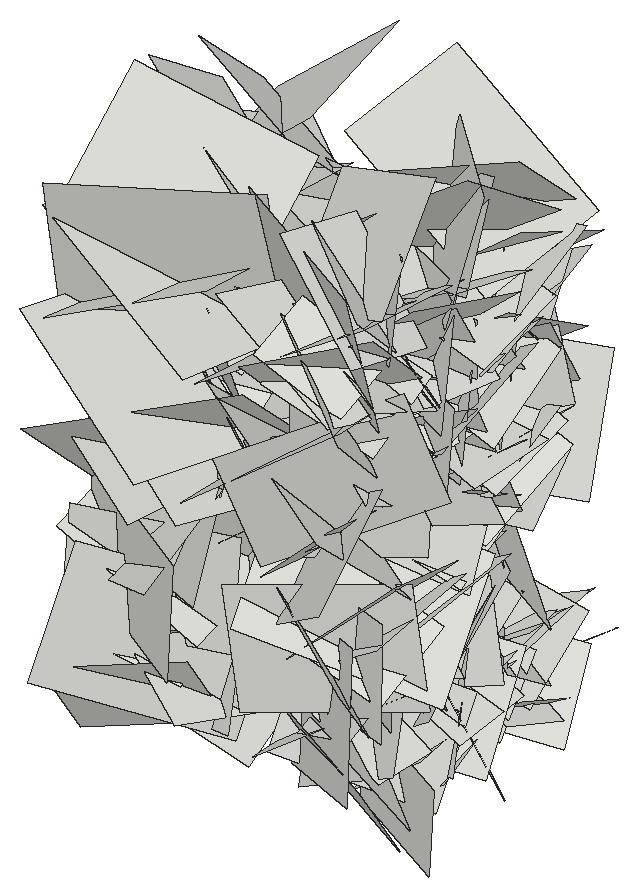
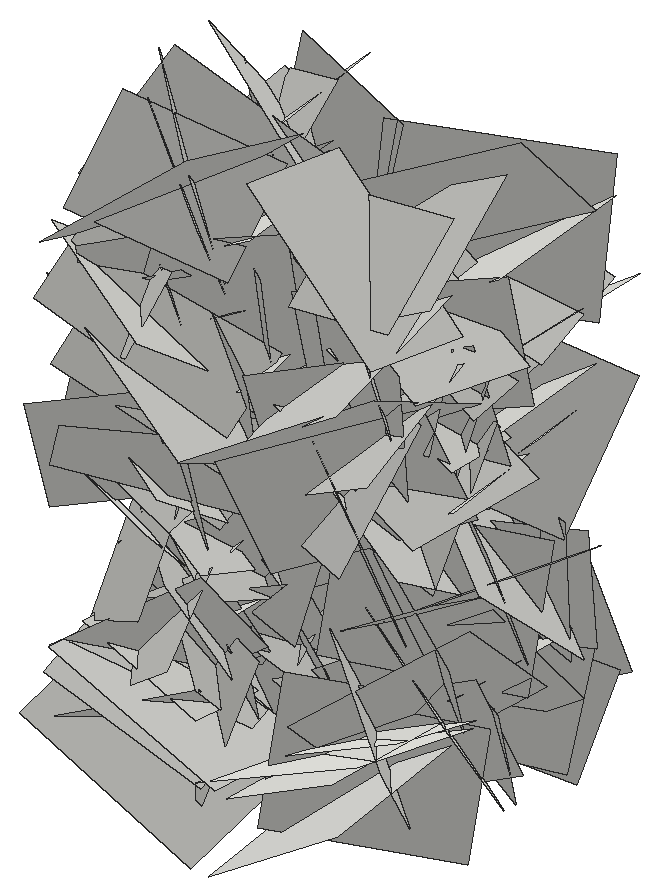
# SketchUp Ruby script. Lengths in inches.
U = 1.inch
M = Sketchup.active_model
def pt(a) = Geom::Point3d.new(a.map { |v| v * U })
def face(e, loops, mat)
  f = e.add_face(loops[0].map { |a| pt(a) })
  loops[1..].each { |l| e.add_face(l.map { |a| pt(a) }).erase! }
  f.material = f.back_material = mat if mat
  f
end
# faces: each face lists its corners as indices into pts; further lists are holes
def faces(e, pts, list, mat = nil) = list.each { |f| face(e, (f[0].is_a?(Array) ? f : [f]).map { |l| l.map { |i| pts[i] } }, mat) }
# xy, xz, yz: faces in a plane at the given z, y or x. An outline is a flat list of corners, or four numbers for a rectangle; further outlines are holes
def ring(l) = l.size == 4 ? [[l[0], l[1]], [l[2], l[1]], [l[2], l[3]], [l[0], l[3]]] : l.each_slice(2).to_a
def flat(e, list, mat, &to3) = list.each { |f| face(e, (f[0].is_a?(Array) ? f : [f]).map { |l| ring(l).map { |u, v| to3.(u, v) } }, mat) }
def xy(e, z, list, mat = nil) = flat(e, list, mat) { |x, y| [x, y, z] }
def xz(e, y, list, mat = nil) = flat(e, list, mat) { |x, z| [x, y, z] }
def yz(e, x, list, mat = nil) = flat(e, list, mat) { |y, z| [x, y, z] }
def lines(e, pts, list) = list.each { |a, b| e.add_line(pt(pts[a]), pt(pts[b])) }
# prism: a flat outline (further loops are holes) pulled along v
def prism(e, loops, v, mat = nil)
  f = face(e, loops, mat); d = Geom::Vector3d.new(v.map { |x| x * U })
  f.pushpull(f.normal.samedirection?(d) ? d.length : -d.length)
end
def box(e, o, s, mat = nil) = prism(e, [[o, [o[0] + s[0], o[1], o[2]], [o[0] + s[0], o[1] + s[1], o[2]], [o[0], o[1] + s[1], o[2]]]], [0, 0, s[2]], mat)
def at(x, y, z, deg = 0) = Geom::Transformation.translation(pt([x, y, z])) * Geom::Transformation.rotation(ORIGIN, Z_AXIS, deg.degrees)
def axes(o, x, y, z) = Geom::Transformation.new([*x, 0, *y, 0, *z, 0, *pt(o).to_a, 1])
def part(name) = M.definitions.add(name)
# library, detail: a bought-in or finely detailed component or shape, given as its bounding box
def library(name, o, s) = part(name).tap { |d| box(d.entities, o, s) }
def detail(e, o, s) = box(e.add_group.entities, o, s)
def put(e, d, t, mat = nil) = e.add_instance(d, t).tap { |i| i.material = mat if mat }
def group(e, t, mat = nil) = e.add_group.tap { |g| g.transformation = t; g.material = mat if mat }.entities
root = M.entities
c1 = part("Component\#6")
p = [[0.01,0,0],[0,3.24,4.54],[4.32,3.24,4.54],[4.33,0,0]]
faces(c1.entities,p,[[0,1,2,3]])
put(root,c1,axes([400.91,196.19,13.89],[-0.03711,0.95345,-0.08325],[0.1071,-0.07916,-0.94908],[1.00884,0.04348,0.09769]))
put(root,c1,axes([404.88,198.53,13.8],[0.10676,-0.41647,0.70694],[0.09382,0.7136,0.40779],[-0.86465,0.02601,0.13154]))
put(root,c1,axes([404.88,201.03,8.02],[0.03451,-0.61291,-0.20918],[-0.0475,-0.21108,0.61149],[-0.68484,-0.01625,-0.05296]))
put(root,c1,axes([404.88,199.53,17.66],[0.07108,0.22718,0.77768],[0.14032,0.76678,-0.23541],[-0.84726,0.14605,0.02626]))
put(root,c1,axes([404.88,196.1,5.28],[0.08762,-0.56519,-0.39893],[-0.0287,-0.4041,0.56691],[-0.73275,-0.05175,-0.06991]))
put(root,c1,axes([400.91,192.44,8.79],[-0.05887,1.04295,0.25043],[0.00297,0.2509,-1.04431],[1.13694,0.05335,0.0157]))
put(root,c1,axes([400.91,193.71,0.46],[0.00413,-0.52236,0.7551],[0.18121,0.74232,0.51263],[0.95624,-0.13842,-0.10041]))
put(root,c1,axes([400.91,195.28,4.79],[0.03702,0.87634,0.85063],[-0.28559,0.83554,-0.84973],[1.26267,0.16329,-0.21713]))
put(root,c1,axes([400.91,203.91,5.3125],[0.18463,-0.58129,-0.78091],[-0.13848,-0.80009,0.56643],[1.02258,-0.00339,0.2177]))
put(root,c1,axes([400.91,198.93,5.125],[0.08676,0.85287,0.14934],[0.16568,0.13299,-0.84515],[0.90272,-0.10637,0.14076]))
put(root,c1,axes([400.91,198.84,9.75],[-0.24721,-0.9594,-0.88495],[-0.06038,-0.89063,0.98057],[1.38221,-0.2105,-0.11544]))
put(root,c1,axes([400.91,202.1,18.26],[-0.1919,-1.13475,-0.09678],[0.16378,-0.12156,1.13628],[1.19604,-0.16542,-0.17113]))
put(root,c1,axes([404.88,194.11,10.49],[0.01019,-0.66626,0.06574],[0.1187,0.06642,0.65679],[-0.69967,0.00157,0.11238]))
put(root,c1,axes([400.91,200.51,5.45],[-0.07717,-0.59417,-0.91785],[0.09928,-0.91989,0.58806],[1.15472,0.03938,-0.1119]))
put(root,c1,axes([400.91,205.24,14.9],[-0.1168,-0.46047,-1.13614],[-0.0362,-1.13913,0.465],[1.29896,-0.07315,-0.0892]))
put(root,c1,axes([400.91,194.25,1.05],[0.1707,-0.55728,0.79671],[-0.04122,0.80323,0.5697],[1.02978,0.12452,-0.10926]))
put(root,c1,axes([400.91,194.35,10.5],[-0.1187,0.07765,-1.12146],[0.14385,-1.11784,-0.09095],[1.18288,0.14373,-0.10148]))
put(root,c1,axes([400.91,197.36,24.8],[-0.09794,1.0389,-0.68546],[-0.01654,-0.68826,-1.04104],[1.31923,0.0685,-0.06394]))
put(root,c1,axes([404.88,199.74,12.37],[0.13977,-0.41949,-0.41774],[-0.0557,-0.43458,0.41982],[-0.62506,-0.05508,-0.13082]))
put(root,c1,axes([404.88,199.42,15.6],[0.03605,-0.49998,-0.38134],[0.14474,-0.36691,0.49324],[-0.65063,-0.10932,0.0886]))
put(root,c1,axes([400.91,200.08,24.34],[0.03463,0.75517,-0.67877],[0.20748,-0.67107,-0.73718],[1.05612,0.10708,0.16708]))
put(root,c1,axes([400.91,199.09,16.39],[0.13116,-1.14374,0.05938],[-0.13174,0.04596,1.1443],[1.20683,0.12933,0.11846]))
put(root,c1,axes([400.91,192.66,5.0625],[0.03803,0.06475,1.02957],[0.25075,1.00223,-0.07127],[1.06436,-0.23842,-0.02]))
put(root,c1,axes([400.91,196.53,2.03],[0.14871,0.38131,0.94323],[0.09041,0.94439,-0.39446],[1.07463,-0.13222,-0.09734]))
put(root,c1,axes([400.91,200.2,14.91],[0.20407,-0.96139,-0.18597],[0.07393,-0.17559,0.97991],[1.03533,0.20204,-0.03331]))
put(root,c1,axes([400.91,198.375,11.05],[-0.00636,-0.47599,-1.14741],[-0.03555,-1.14695,0.47597],[1.31628,-0.03327,0.00731]))
put(root,c1,axes([400.91,202.25,12.93],[-0.19135,-1.27912,0.12446],[0.2118,0.09622,1.27869],[1.34571,-0.19703,-0.18355]))
put(root,c1,axes([400.91,197.86,18.23],[0.19608,0.2602,-1.0463],[-0.01915,-1.06069,-0.26697],[1.14269,-0.06243,0.17507]))
put(root,c1,axes([400.91,197.84,4.84],[0.11369,-0.36766,-0.96616],[0.19069,-0.94989,0.38144],[1.07906,0.2066,0.03439]))
put(root,c1,axes([400.91,200.375,7.61],[0.26418,-0.51362,-0.84712],[0.05211,-0.86603,0.53955],[1.04881,0.1724,0.18657]))
put(root,c1,axes([400.91,203.04,12.11],[0.14841,-0.94408,-0.5752],[0.05434,-0.57362,0.95398],[1.17058,0.14632,0.02864]))
put(root,c1,axes([400.91,199.56,18.73],[0.07364,1.07871,-0.62029],[-0.05176,-0.61841,-1.08091],[1.31797,-0.08456,-0.00779]))
put(root,c1,axes([400.91,204.42,20.53],[0.1154,-1.25003,-0.28156],[-0.14973,-0.29256,1.24425],[1.34995,0.07441,0.16208]))
put(root,c1,axes([400.91,195.93,15.54],[0.04965,0.25406,1.2028],[0.02984,1.20314,-0.25523],[1.30276,-0.03724,-0.03999]))
put(root,c1,axes([400.91,198.85,12.57],[0.15345,0.48368,1.12599],[-0.09378,1.13498,-0.47617],[1.29562,0.02486,-0.16783]))
put(root,c1,axes([400.91,200.7,5.85],[0.20906,1.0682,-0.14016],[0.07965,-0.15578,-1.08152],[1.13921,-0.18514,0.10133]))
put(root,c1,axes([400.91,194.09,6.34],[0.25898,1.07168,-0.21064],[-0.01285,-0.21318,-1.09862],[1.15764,-0.24212,0.03493]))
put(root,c1,axes([400.91,192.7,21.39],[0.08893,0.79245,0.9015],[0.06254,0.89988,-0.79652],[1.27076,-0.09974,-0.02389]))
put(root,c1,axes([400.91,199.38,-0.0625],[0.15183,-0.50198,1.07326],[0.00307,1.08122,0.50532],[1.25594,0.05804,-0.13098]))
put(root,c1,axes([400.91,200.25,4.79],[0.06637,1.27776,-0.24675],[-0.01199,-0.2465,-1.2793],[1.3794,-0.06362,0.00075]))
put(root,c1,axes([400.91,192.73,15.73],[0.12897,1.2724,-0.23633],[-0.08155,-0.22984,-1.27707],[1.36939,-0.13352,-0.05379]))
put(root,c1,axes([400.91,200.21,21.54],[0.14018,1.21556,-0.55877],[-0.14242,-0.54659,-1.22085],[1.41094,-0.17594,-0.06772]))
put(root,c1,axes([400.91,190.45,18.05],[0.16537,1.24759,-0.14593],[-0.05265,-0.14081,-1.25691],[1.33042,-0.16065,-0.0316]))
put(root,c1,axes([400.91,190.86,3.39],[0.21383,0.32739,1.20741],[-0.09698,1.22359,-0.31649],[1.32251,0.03679,-0.21843]))
put(root,c1,axes([400.91,195.52,16.87],[0.17814,-1.09516,0.21581],[0.19304,0.24222,1.08736],[1.16734,0.12707,-0.21275]))
put(root,c1,axes([400.91,201.79,17.38],[0.19939,0.73728,-1.06028],[-0.09629,-1.06126,-0.75408],[1.36551,-0.18249,0.10164]))
put(root,c1,axes([400.91,196.26,4.8],[0.10051,-0.43998,1.12809],[0.21352,1.12151,0.42048],[1.26562,-0.15427,-0.16053]))
put(root,c1,axes([400.91,191.67,21.5],[0.0579,1.33618,-0.15223],[0.05318,-0.15428,-1.33612],[1.42453,-0.04855,0.05606]))
put(root,c1,axes([400.91,198.6875,16.83],[0.02201,1.26014,0.56955],[0.0456,0.56875,-1.25994],[1.46513,-0.03663,0.03065]))
put(root,c1,axes([400.91,196.95,13.22],[0.12152,0.35472,1.26895],[0.01769,1.27325,-0.35743],[1.39654,-0.047,-0.10589]))
put(root,c1,axes([400.91,197.84,15.77],[0.08558,0.66637,-1.22765],[0.01617,-1.23004,-0.66667],[1.48057,-0.02508,0.07824]))
put(root,c1,axes([400.91,193.34,3.5],[0.3285,0.68164,0.95344],[0.04901,0.97833,-0.71446],[1.2414,-0.219,-0.22409]))
put(root,c1,axes([400.91,192.59,17.15],[0.08597,-0.32374,1.28455],[0.18245,1.27862,0.31138],[1.3923,-0.14756,-0.12012]))
put(root,c1,axes([400.91,199.09,4.9],[0.11121,1.25407,0.182],[0.25083,0.16003,-1.23904],[1.31962,-0.1361,0.22018]))
put(root,c1,axes([400.91,194.4,9.86],[0.11876,-1.04596,0.91618],[0.1474,0.92297,1.03671],[1.46651,-0.00807,-0.1784]))
put(root,c1,axes([400.91,202.95,19.72],[0.19445,-0.3512,-1.29554],[0.25274,-1.27827,0.38028],[1.40021,0.2795,0.11127]))
put(root,c1,axes([414.68,202.95,19.72],[-0.19445,-0.3512,-1.29554],[-0.25274,-1.27827,0.38028],[-1.40021,0.2795,0.11127]))
put(root,c1,axes([414.68,194.4,9.86],[-0.11876,-1.04596,0.91618],[-0.1474,0.92297,1.03671],[-1.46651,-0.00807,-0.1784]))
put(root,c1,axes([414.68,199.09,4.9],[-0.11121,1.25407,0.182],[-0.25083,0.16003,-1.23904],[-1.31962,-0.1361,0.22018]))
put(root,c1,axes([414.68,192.59,17.15],[-0.08597,-0.32374,1.28455],[-0.18245,1.27862,0.31138],[-1.3923,-0.14756,-0.12012]))
put(root,c1,axes([414.68,193.34,3.5],[-0.3285,0.68164,0.95344],[-0.04901,0.97833,-0.71446],[-1.2414,-0.219,-0.22409]))
put(root,c1,axes([414.68,197.84,15.77],[-0.08558,0.66637,-1.22765],[-0.01617,-1.23004,-0.66667],[-1.48057,-0.02508,0.07824]))
put(root,c1,axes([414.68,196.95,13.22],[-0.12152,0.35472,1.26895],[-0.01769,1.27325,-0.35743],[-1.39654,-0.047,-0.10589]))
put(root,c1,axes([414.68,198.6875,16.83],[-0.02201,1.26014,0.56955],[-0.0456,0.56875,-1.25994],[-1.46513,-0.03663,0.03065]))
put(root,c1,axes([414.68,191.67,21.5],[-0.0579,1.33618,-0.15223],[-0.05318,-0.15428,-1.33612],[-1.42453,-0.04855,0.05606]))
put(root,c1,axes([414.68,196.26,4.8],[-0.10051,-0.43998,1.12809],[-0.21352,1.12151,0.42048],[-1.26562,-0.15427,-0.16053]))
put(root,c1,axes([414.68,201.79,17.38],[-0.19939,0.73728,-1.06028],[0.09629,-1.06126,-0.75408],[-1.36551,-0.18249,0.10164]))
put(root,c1,axes([414.68,195.52,16.87],[-0.17814,-1.09516,0.21581],[-0.19304,0.24222,1.08736],[-1.16734,0.12707,-0.21275]))
put(root,c1,axes([414.68,190.86,3.39],[-0.21383,0.32739,1.20741],[0.09698,1.22359,-0.31649],[-1.32251,0.03679,-0.21843]))
put(root,c1,axes([414.68,190.45,18.05],[-0.16537,1.24759,-0.14593],[0.05265,-0.14081,-1.25691],[-1.33042,-0.16065,-0.0316]))
put(root,c1,axes([414.68,200.21,21.54],[-0.14018,1.21556,-0.55877],[0.14242,-0.54659,-1.22085],[-1.41094,-0.17594,-0.06772]))
put(root,c1,axes([414.68,192.73,15.73],[-0.12897,1.2724,-0.23633],[0.08155,-0.22984,-1.27707],[-1.36939,-0.13352,-0.05379]))
put(root,c1,axes([414.68,200.25,4.79],[-0.06637,1.27776,-0.24675],[0.01199,-0.2465,-1.2793],[-1.3794,-0.06362,0.00075]))
put(root,c1,axes([414.68,199.38,-0.0625],[-0.15183,-0.50198,1.07326],[-0.00307,1.08122,0.50532],[-1.25594,0.05804,-0.13098]))
put(root,c1,axes([414.68,192.7,21.39],[-0.08893,0.79245,0.9015],[-0.06254,0.89988,-0.79652],[-1.27076,-0.09974,-0.02389]))
put(root,c1,axes([414.68,194.09,6.34],[-0.25898,1.07168,-0.21064],[0.01285,-0.21318,-1.09862],[-1.15764,-0.24212,0.03493]))
put(root,c1,axes([414.68,200.7,5.85],[-0.20906,1.0682,-0.14016],[-0.07965,-0.15578,-1.08152],[-1.13921,-0.18514,0.10133]))
put(root,c1,axes([414.68,198.85,12.57],[-0.15345,0.48368,1.12599],[0.09378,1.13498,-0.47617],[-1.29562,0.02486,-0.16783]))
put(root,c1,axes([414.68,195.93,15.54],[-0.04965,0.25406,1.2028],[-0.02984,1.20314,-0.25523],[-1.30276,-0.03724,-0.03999]))
put(root,c1,axes([414.68,204.42,20.53],[-0.1154,-1.25003,-0.28156],[0.14973,-0.29256,1.24425],[-1.34995,0.07441,0.16208]))
put(root,c1,axes([414.68,199.56,18.73],[-0.07364,1.07871,-0.62029],[0.05176,-0.61841,-1.08091],[-1.31797,-0.08456,-0.00779]))
put(root,c1,axes([414.68,203.04,12.11],[-0.14841,-0.94408,-0.5752],[-0.05434,-0.57362,0.95398],[-1.17058,0.14632,0.02864]))
put(root,c1,axes([414.68,200.375,7.61],[-0.26418,-0.51362,-0.84712],[-0.05211,-0.86603,0.53955],[-1.04881,0.1724,0.18657]))
put(root,c1,axes([414.68,197.84,4.84],[-0.11369,-0.36766,-0.96616],[-0.19069,-0.94989,0.38144],[-1.07906,0.2066,0.03439]))
put(root,c1,axes([414.68,197.86,18.23],[-0.19608,0.2602,-1.0463],[0.01915,-1.06069,-0.26697],[-1.14269,-0.06243,0.17507]))
put(root,c1,axes([414.68,202.25,12.93],[0.19135,-1.27912,0.12446],[-0.2118,0.09622,1.27869],[-1.34571,-0.19703,-0.18355]))
put(root,c1,axes([414.68,198.375,11.05],[0.00636,-0.47599,-1.14741],[0.03555,-1.14695,0.47597],[-1.31628,-0.03327,0.00731]))
put(root,c1,axes([414.68,200.2,14.91],[-0.20407,-0.96139,-0.18597],[-0.07393,-0.17559,0.97991],[-1.03533,0.20204,-0.03331]))
put(root,c1,axes([414.68,196.53,2.03],[-0.14871,0.38131,0.94323],[-0.09041,0.94439,-0.39446],[-1.07463,-0.13222,-0.09734]))
put(root,c1,axes([414.68,192.66,5.0625],[-0.03803,0.06475,1.02957],[-0.25075,1.00223,-0.07127],[-1.06436,-0.23842,-0.02]))
put(root,c1,axes([414.68,199.09,16.39],[-0.13116,-1.14374,0.05938],[0.13174,0.04596,1.1443],[-1.20683,0.12933,0.11846]))
put(root,c1,axes([414.68,200.08,24.34],[-0.03463,0.75517,-0.67877],[-0.20748,-0.67107,-0.73718],[-1.05612,0.10708,0.16708]))
put(root,c1,axes([410.71,199.42,15.6],[-0.03605,-0.49998,-0.38134],[-0.14474,-0.36691,0.49324],[0.65063,-0.10932,0.0886]))
put(root,c1,axes([410.71,199.74,12.37],[-0.13977,-0.41949,-0.41774],[0.0557,-0.43458,0.41982],[0.62506,-0.05508,-0.13082]))
put(root,c1,axes([414.68,197.36,24.8],[0.09794,1.0389,-0.68546],[0.01654,-0.68826,-1.04104],[-1.31923,0.0685,-0.06394]))
put(root,c1,axes([414.68,194.35,10.5],[0.1187,0.07765,-1.12146],[-0.14385,-1.11784,-0.09095],[-1.18288,0.14373,-0.10148]))
put(root,c1,axes([414.68,194.25,1.05],[-0.1707,-0.55728,0.79671],[0.04122,0.80323,0.5697],[-1.02978,0.12452,-0.10926]))
put(root,c1,axes([414.68,205.24,14.9],[0.1168,-0.46047,-1.13614],[0.0362,-1.13913,0.465],[-1.29896,-0.07315,-0.0892]))
put(root,c1,axes([414.68,200.51,5.45],[0.07717,-0.59417,-0.91785],[-0.09928,-0.91989,0.58806],[-1.15472,0.03938,-0.1119]))
put(root,c1,axes([410.71,194.11,10.49],[-0.01019,-0.66626,0.06574],[-0.1187,0.06642,0.65679],[0.69967,0.00157,0.11238]))
put(root,c1,axes([414.68,202.1,18.26],[0.1919,-1.13475,-0.09678],[-0.16378,-0.12156,1.13628],[-1.19604,-0.16542,-0.17113]))
put(root,c1,axes([414.68,198.84,9.75],[0.24721,-0.9594,-0.88495],[0.06038,-0.89063,0.98057],[-1.38221,-0.2105,-0.11544]))
put(root,c1,axes([414.68,198.93,5.125],[-0.08676,0.85287,0.14934],[-0.16568,0.13299,-0.84515],[-0.90272,-0.10637,0.14076]))
put(root,c1,axes([414.68,203.91,5.3125],[-0.18463,-0.58129,-0.78091],[0.13848,-0.80009,0.56643],[-1.02258,-0.00339,0.2177]))
put(root,c1,axes([414.68,195.28,4.79],[-0.03702,0.87634,0.85063],[0.28559,0.83554,-0.84973],[-1.26267,0.16329,-0.21713]))
put(root,c1,axes([414.68,193.71,0.46],[-0.00413,-0.52236,0.7551],[-0.18121,0.74232,0.51263],[-0.95624,-0.13842,-0.10041]))
put(root,c1,axes([414.68,192.44,8.79],[0.05887,1.04295,0.25043],[-0.00297,0.2509,-1.04431],[-1.13694,0.05335,0.0157]))
put(root,c1,axes([410.71,196.1,5.28],[-0.08762,-0.56519,-0.39893],[0.0287,-0.4041,0.56691],[0.73275,-0.05175,-0.06991]))
put(root,c1,axes([410.71,199.53,17.66],[-0.07108,0.22718,0.77768],[-0.14032,0.76678,-0.23541],[0.84726,0.14605,0.02626]))
put(root,c1,axes([410.71,201.03,8.02],[-0.03451,-0.61291,-0.20918],[0.0475,-0.21108,0.61149],[0.68484,-0.01625,-0.05296]))
put(root,c1,axes([410.71,198.53,13.8],[-0.10676,-0.41647,0.70694],[-0.09382,0.7136,0.40779],[0.86465,0.02601,0.13154]))
put(root,c1,axes([414.68,196.19,13.89],[0.03711,0.95345,-0.08325],[-0.1071,-0.07916,-0.94908],[-1.00884,0.04348,0.09769]))
put(root,c1,axes([414.68,197.24,20.32],[-0.11105,0.4932,0.81979],[0.10012,0.82599,-0.48487],[-1.00916,0.02768,-0.13831]))
put(root,c1,axes([410.71,202.56,19.21],[0.06396,-0.26998,-0.58675],[-0.04641,-0.58965,0.26682],[0.68306,-0.01478,0.07307]))
put(root,c1,axes([410.71,199.64,2.06],[-0.21894,0.61345,0.59822],[0.01858,0.61825,-0.62794],[0.90807,0.13525,0.15708]))
put(root,c1,axes([414.68,196.07,8.125],[-0.08332,-0.69698,-0.457],[-0.10667,-0.44773,0.70016],[-0.87699,0.12068,-0.04174]))
put(root,c1,axes([410.71,190.79,19.57],[0.04866,0.55121,0.30162],[0.00575,0.30207,-0.55285],[0.66601,-0.04288,-0.01726]))
put(root,c1,axes([410.71,195.85,11.01],[-0.15114,0.73817,0.19544],[0.07767,0.21113,-0.74396],[0.80568,0.11812,0.10838]))
put(root,c1,axes([414.68,202.76,13.17],[0.11284,-1.03894,-0.17524],[-0.03066,-0.17895,1.04335],[-1.11641,-0.1001,-0.04636]))
put(root,c1,axes([414.68,189.31,11.46],[-0.01967,0.80876,0.77653],[0.21901,0.76581,-0.79265],[-1.16812,0.12996,-0.16169]))
put(root,c1,axes([410.71,193.57,4.75],[0.0218,0.6351,0.02763],[0.03876,0.02642,-0.63443],[0.67273,-0.0221,0.03566]))
put(root,c1,axes([414.68,199.68,18.17],[0.10811,0.81171,0.57509],[-0.11351,0.5837,-0.80488],[-1.04835,0.0205,0.14645]))
put(root,c1,axes([410.71,202.9,8.46],[-0.28421,-0.45126,-0.90988],[-0.10984,-0.92399,0.48879],[1.07096,-0.21452,-0.19133]))
put(root,c1,axes([410.71,193.91,15.9375],[0.03263,0.61645,-0.26034],[-0.02336,-0.25954,-0.61716],[0.70894,-0.03692,-0.00835]))
put(root,c1,axes([410.71,192.26,20.51],[-0.14395,0.6641,-0.62024],[-0.10915,-0.63433,-0.65665],[0.95701,0.02754,-0.16819]))
put(root,c1,axes([410.71,199.23,1.1],[-0.00098,-0.71414,-0.15761],[-0.04174,-0.15733,0.71311],[0.77408,-0.00939,0.03826]))
put(root,c1,axes([410.71,196.5625,6.92],[0.07674,-0.09799,-0.6482],[-0.03176,-0.65195,0.09521],[0.69417,-0.019,0.07601]))
put(root,c1,axes([410.71,198.91,12.75],[-0.15355,-0.10183,1.00426],[-0.21738,0.99636,0.07145],[1.04766,0.19182,0.16201]))
put(root,c1,axes([410.71,195.68,15.75],[0.06715,-0.51242,0.33521],[0.05381,0.34023,0.51051],[0.64683,0.02489,-0.07727]))
put(root,c1,axes([410.71,200.4375,8.06],[-0.17377,0.75884,-0.49804],[-0.05898,-0.51355,-0.76415],[0.96033,0.10576,-0.13705]))
put(root,c1,axes([410.71,199.6875,17.84],[0.07891,0.44569,0.39814],[0.07493,0.39183,-0.45185],[0.62903,-0.10259,0.00388]))
put(root,c1,axes([410.71,200.03,9.27],[-0.00412,-0.60297,0.30435],[0.07057,0.30253,0.60022],[0.71247,-0.03345,-0.05769]))
put(root,c1,axes([410.71,192.95,10.8],[0.02962,0.02518,0.78508],[-0.12702,0.77652,-0.02064],[0.82287,0.11896,-0.03145]))
put(root,c1,axes([414.68,199.37,10.67],[0.09558,-1.01864,0.46326],[0.13943,0.47118,1.01047],[-1.17795,-0.02688,0.1572]))
put(root,c1,axes([410.71,198.38,4.95],[-0.02223,0.32868,-0.55446],[0.17267,-0.53404,-0.32274],[0.66105,0.15055,0.06565]))
put(root,c1,axes([410.71,192.04,10.01],[-0.12172,0.5206,-0.6372],[0.01939,-0.6416,-0.52749],[0.87198,0.08694,-0.07722]))
put(root,c1,axes([410.71,202.51,19.98],[0.06792,0.48446,-0.5602],[-0.10116,-0.55221,-0.48846],[0.77852,-0.11402,-0.01459]))
put(root,c1,axes([414.68,195.86,16.68],[-0.06531,-0.43873,0.684],[-0.07025,0.68639,0.43429],[-0.8585,-0.02279,-0.08757]))
put(root,c1,axes([410.71,202.74,-0.14],[0.03158,-0.64507,0.25861],[0.01592,0.25938,0.64528],[0.73651,0.02205,-0.02503]))
put(root,c1,axes([414.68,192.22,20.81],[-0.00161,0.62306,-0.59539],[-0.0785,-0.59329,-0.62067],[-0.91013,0.05007,0.05459]))
put(root,c1,axes([410.71,197.35,3.52],[0.03443,0.41092,0.66217],[-0.08038,0.66126,-0.40665],[0.82215,0.04744,-0.06748]))
put(root,c1,axes([410.71,195.99,4.23],[-0.18601,0.0566,0.88651],[0.05201,0.90288,-0.04793],[0.94017,-0.03875,0.17804]))
put(root,c1,axes([414.68,198.67,11.97],[0.07539,0.76068,0.50866],[-0.0723,0.51318,-0.75791],[-0.96729,0.02092,0.0963]))
put(root,c1,axes([410.71,195.9375,9.16],[0.07841,0.69576,-0.29748],[-0.09095,-0.28926,-0.69787],[0.79692,-0.10147,-0.05038]))
put(root,c1,axes([414.68,195.4375,18.11],[-0.16874,-0.51977,-0.57708],[0.05885,-0.59519,0.52076],[-0.82114,0.06415,0.15591]))
put(root,c1,axes([414.68,196.17,12.88],[0.06274,0.02618,0.84664],[-0.15393,0.83645,-0.01571],[-0.88457,-0.1437,0.06278]))
put(root,c1,axes([414.68,193.46,10.77],[-0.10152,0.90556,-0.18731],[0.17799,-0.16815,-0.89879],[-0.96391,-0.12642,-0.14624]))
put(root,c1,axes([410.71,200.82,0.59],[0.02153,-0.73416,-0.35765],[-0.0933,-0.35764,0.72915],[0.8606,-0.02041,0.08799]))
put(root,c1,axes([414.68,195.73,16.63],[0.01219,-0.78698,0.32297],[-0.05977,0.32158,0.78561],[-0.89973,-0.03203,-0.04781]))
put(root,c1,axes([414.68,196.375,20.79],[0.12547,0.87042,-0.10702],[-0.18806,-0.08199,-0.86307],[-0.91037,0.1369,0.16354]))
put(root,c1,axes([414.68,200.05,13.66],[-0.07814,0.81604,-0.08962],[0.02759,-0.08761,-0.81916],[-0.86976,-0.0761,-0.01794]))
put(root,c1,axes([414.68,198.3125,4.47],[0.08144,0.93817,-0.09306],[0.01009,-0.09413,-0.94116],[-0.99929,0.07551,-0.01709]))
put(root,c1,axes([414.68,200.41,3.58],[0.05776,-0.87144,-0.04483],[-0.06577,-0.04867,0.87073],[-0.92261,-0.05109,-0.06488]))
put(root,c1,axes([414.68,195.95,14.86],[0.17446,0.9838,0.62037],[0.19333,0.59697,-0.99508],[-1.2176,0.23574,-0.06911]))
put(root,c1,axes([414.68,194.43,21.03],[0.18864,1.08922,-0.2367],[0.12278,-0.25647,-1.09312],[-1.17512,0.14806,-0.15221]))
put(root,c1,axes([410.71,200.69,6.875],[-0.16125,-0.91938,-0.30199],[-0.04119,-0.29965,0.93182],[1.02494,-0.15668,-0.01006]))
put(root,c1,axes([414.68,193.09,19.46],[-0.07295,0.25641,0.83596],[0.12348,0.83376,-0.24615],[-0.9186,0.09171,-0.09948]))
put(root,c1,axes([414.68,196.25,20.97],[-0.03433,0.46285,-0.75346],[0.09275,-0.74858,-0.46362],[-0.93272,-0.09148,-0.01837]))
put(root,c1,axes([410.71,193.9,23.36],[0.05376,0.55183,-0.55937],[-0.04326,-0.55793,-0.55411],[0.83178,-0.06469,0.00734]))
put(root,c1,axes([414.68,193.92,18.08],[0.13809,0.41624,-1.10581],[0.27382,-1.09563,-0.38198],[-1.22215,-0.19844,-0.21052]))
put(root,c1,axes([414.68,202.38,16.09],[0.07402,-0.92988,-0.45649],[0.17154,-0.44211,0.92536],[-1.08456,-0.13339,0.1152]))
put(root,c1,axes([410.71,201.99,11.3125],[-0.07595,0.62186,-0.76254],[-0.14567,-0.76339,-0.60964],[1.03278,-0.06194,-0.14206]))
put(root,c1,axes([410.71,202.11,15.27],[0.00741,-0.76642,-0.19435],[0.02033,-0.19414,0.76626],[0.83787,0.01149,-0.01688]))
put(root,c1,axes([414.68,195.27,-1.16],[0.10176,-0.07093,0.82892],[-0.16666,0.81783,0.08819],[-0.86597,-0.16573,0.08043]))
put(root,c1,axes([414.68,196.11,19.5625],[0.1708,0.27531,1.11719],[0.21419,1.10379,-0.30115],[-1.2007,0.23607,0.1052]))
put(root,c1,axes([410.71,200.46,4.14],[0.03987,0.66432,-0.22968],[0.12809,-0.2327,-0.65325],[0.73398,0.00452,0.12648]))
put(root,c1,axes([414.68,200.85,9.74],[-0.02518,0.49854,0.49521],[-0.19267,0.47427,-0.48618],[-0.7195,-0.14445,0.11286]))
put(root,c1,axes([410.71,192.1875,23.6],[0.04344,0.89705,-0.17333],[-0.1764,-0.16328,-0.88435],[0.95226,-0.07116,-0.15591]))
